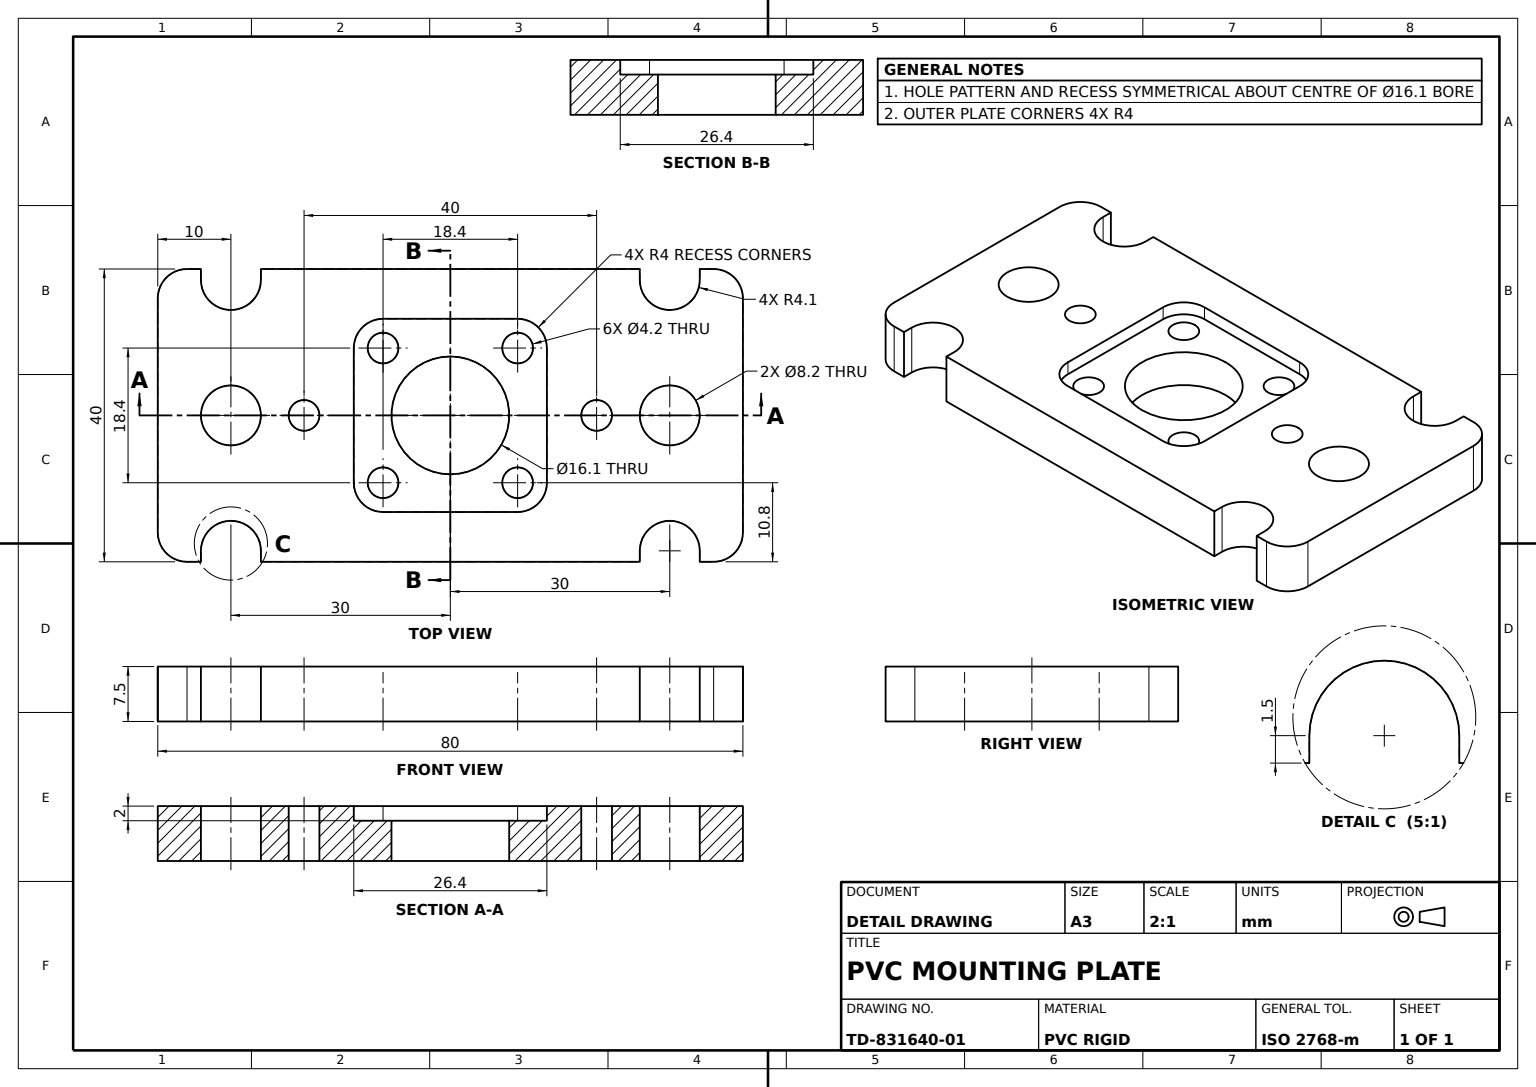
solid
v1 (-40,7.5,-16)
v2 (-40,0,-16)
e1 v1 v2 LINE
v3 (-36,7.5,-20)
e2 v3 v1 CIRCLE(AX(P(-36,7.5,-16),D(0,1,0),D(0,0,-1)),4)
v4 (-36,0,-20)
e3 v3 v4 LINE
e4 v4 v2 CIRCLE(AX(P(-36,0,-16),D(0,1,0),D(0,0,-1)),4)
face CYL(AX(P(-36,7.5,-16),D(0,-1,0),D(0,0,-1)),4) [-e1 -e2 e3 e4]
v5 (36,7.5,-20)
v6 (36,0,-20)
e5 v5 v6 LINE
v7 (40,7.5,-16)
e6 v7 v5 CIRCLE(AX(P(36,7.5,-16),D(0,1,0),D(0,0,1)),4)
v8 (40,0,-16)
e7 v7 v8 LINE
e8 v8 v6 CIRCLE(AX(P(36,0,-16),D(0,1,0),D(0,0,1)),4)
face CYL(AX(P(36,7.5,-16),D(0,-1,0),D(0,0,-1)),4) [-e5 -e6 e7 e8]
v9 (-20,7.5,2.1)
v10 (-20,7.5,-2.1)
e9 v9 v10 CIRCLE(AX(P(-20,7.5,0),D(0,1,0),D(0,0,1)),2.1)
v11 (-20,0,-2.1)
e10 v10 v11 LINE
v12 (-20,0,2.1)
e11 v12 v11 CIRCLE(AX(P(-20,0,0),D(0,1,0),D(0,0,1)),2.1)
e12 v9 v12 LINE
face CYL(AX(P(-20,7.5,0),D(0,-1,0),D(0,0,-1)),2.1) rev [e9 e10 -e11 -e12]
v13 (-9.2,0,-11.3)
v14 (-9.2,5.5,-11.3)
e13 v13 v14 LINE
v15 (-9.2,0,-7.1)
e14 v13 v15 CIRCLE(AX(P(-9.2,0,-9.2),D(0,-1,0),D(0,0,1)),2.1)
v16 (-9.2,5.5,-7.1)
e15 v15 v16 LINE
e16 v16 v14 CIRCLE(AX(P(-9.2,5.5,-9.2),D(0,1,0),D(0,0,1)),2.1)
face CYL(AX(P(-9.2,-0.001,-9.2),D(0,1,0),D(0,0,1)),2.1) rev [-e13 e14 e15 e16]
v17 (34.1,7.5,-18.5)
v18 (34.1,0,-18.5)
e17 v17 v18 LINE
v19 (25.9,0,-18.5)
e18 v18 v19 CIRCLE(AX(P(30,0,-18.5),D(0,-1,0),D(0,0,1)),4.1)
v20 (25.9,7.5,-18.5)
e19 v20 v19 LINE
e20 v17 v20 CIRCLE(AX(P(30,7.5,-18.5),D(0,-1,0),D(0,0,1)),4.1)
face CYL(AX(P(30,7.5,-18.5),D(0,-1,0),D(0,0,-1)),4.1) rev [e17 e18 -e19 -e20]
v21 (-9.2,0,7.1)
v22 (-9.2,5.5,7.1)
e21 v21 v22 LINE
v23 (-9.2,5.5,11.3)
e22 v22 v23 CIRCLE(AX(P(-9.2,5.5,9.2),D(0,1,0),D(0,0,-1)),2.1)
v24 (-9.2,0,11.3)
e23 v24 v23 LINE
e24 v24 v21 CIRCLE(AX(P(-9.2,0,9.2),D(0,-1,0),D(0,0,1)),2.1)
face CYL(AX(P(-9.2,-0.001,9.2),D(0,1,0),D(0,0,1)),2.1) rev [e21 e22 -e23 e24]
v25 (-34.1,7.5,18.5)
v26 (-34.1,0,18.5)
e25 v25 v26 LINE
v27 (-30,0,14.4)
e26 v26 v27 CIRCLE(AX(P(-30,0,18.5),D(0,-1,0),D(0,0,-1)),4.1)
v28 (-30,7.5,14.4)
e27 v28 v27 LINE
e28 v25 v28 CIRCLE(AX(P(-30,7.5,18.5),D(0,-1,0),D(0,0,-1)),4.1)
face CYL(AX(P(-30,7.5,18.5),D(0,-1,0),D(0,0,-1)),4.1) rev [e25 e26 -e27 -e28]
v29 (0,0,8.05)
v30 (0,5.5,8.05)
e29 v29 v30 LINE
v31 (0,5.5,-8.05)
e30 v30 v31 CIRCLE(AX(P(0,5.5,0),D(0,1,0),D(0,0,1)),8.05)
v32 (0,0,-8.05)
e31 v32 v31 LINE
e32 v32 v29 CIRCLE(AX(P(0,0,0),D(0,-1,0),D(0,0,1)),8.05)
face CYL(AX(P(0,-0.001,0),D(0,1,0),D(0,0,1)),8.05) rev [e29 e30 -e31 e32]
e33 v11 v12 CIRCLE(AX(P(-20,0,0),D(0,1,0),D(0,0,1)),2.1)
e34 v10 v9 CIRCLE(AX(P(-20,7.5,0),D(0,1,0),D(0,0,1)),2.1)
face CYL(AX(P(-20,7.5,0),D(0,-1,0),D(0,0,-1)),2.1) rev [-e33 -e10 e34 e12]
v33 (9.2,0,-11.3)
v34 (9.2,5.5,-11.3)
e35 v33 v34 LINE
v35 (9.2,5.5,-7.1)
e36 v34 v35 CIRCLE(AX(P(9.2,5.5,-9.2),D(0,1,0),D(0,0,-1)),2.1)
v36 (9.2,0,-7.1)
e37 v36 v35 LINE
e38 v36 v33 CIRCLE(AX(P(9.2,0,-9.2),D(0,-1,0),D(0,0,1)),2.1)
face CYL(AX(P(9.2,-0.001,-9.2),D(0,1,0),D(0,0,1)),2.1) rev [e35 e36 -e37 e38]
e39 v33 v36 CIRCLE(AX(P(9.2,0,-9.2),D(0,-1,0),D(0,0,1)),2.1)
e40 v35 v34 CIRCLE(AX(P(9.2,5.5,-9.2),D(0,1,0),D(0,0,-1)),2.1)
face CYL(AX(P(9.2,-0.001,-9.2),D(0,1,0),D(0,0,1)),2.1) rev [-e35 e39 e37 e40]
v37 (36,7.5,20)
v38 (36,0,20)
e41 v37 v38 LINE
v39 (34.1,7.5,20)
e42 v39 v37 LINE
v40 (34.1,0,20)
e43 v39 v40 LINE
e44 v40 v38 LINE
face PLANE(AX(P(34.1,7.5,20),D(0,0,-1),D(-1,0,0))) rev [-e41 -e42 e43 e44]
v41 (-9.2,5.5,-13.2)
v42 (-9.2,7.5,-13.2)
e45 v41 v42 LINE
v43 (-13.2,7.5,-9.2)
e46 v42 v43 CIRCLE(AX(P(-9.2,7.5,-9.2),D(0,1,0),D(0,0,1)),4)
v44 (-13.2,5.5,-9.2)
e47 v44 v43 LINE
e48 v41 v44 CIRCLE(AX(P(-9.2,5.5,-9.2),D(0,1,0),D(0,0,1)),4)
face CYL(AX(P(-9.2,5.5,-9.2),D(0,1,0),D(0,0,1)),4) rev [e45 e46 -e47 -e48]
v45 (9.2,0,7.1)
v46 (9.2,5.5,7.1)
e49 v45 v46 LINE
v47 (9.2,0,11.3)
e50 v45 v47 CIRCLE(AX(P(9.2,0,9.2),D(0,-1,0),D(0,0,1)),2.1)
v48 (9.2,5.5,11.3)
e51 v47 v48 LINE
e52 v48 v46 CIRCLE(AX(P(9.2,5.5,9.2),D(0,1,0),D(0,0,1)),2.1)
face CYL(AX(P(9.2,-0.001,9.2),D(0,1,0),D(0,0,1)),2.1) rev [-e49 e50 e51 e52]
v49 (30,0,4.1)
v50 (30,0,-4.1)
e53 v49 v50 CIRCLE(AX(P(30,0,0),D(0,1,0),D(0,0,-1)),4.1)
v51 (30,7.5,4.1)
e54 v51 v49 LINE
v52 (30,7.5,-4.1)
e55 v51 v52 CIRCLE(AX(P(30,7.5,0),D(0,1,0),D(0,0,-1)),4.1)
e56 v52 v50 LINE
face CYL(AX(P(30,7.5,0),D(0,-1,0),D(0,0,-1)),4.1) rev [-e53 -e54 e55 e56]
e57 v14 v16 CIRCLE(AX(P(-9.2,5.5,-9.2),D(0,1,0),D(0,0,1)),2.1)
e58 v15 v13 CIRCLE(AX(P(-9.2,0,-9.2),D(0,-1,0),D(0,0,1)),2.1)
face CYL(AX(P(-9.2,-0.001,-9.2),D(0,1,0),D(0,0,1)),2.1) rev [e57 -e15 e58 e13]
v53 (9.2,5.5,13.2)
v54 (9.2,7.5,13.2)
e59 v53 v54 LINE
v55 (-9.2,5.5,13.2)
e60 v55 v53 LINE
v56 (-9.2,7.5,13.2)
e61 v55 v56 LINE
e62 v56 v54 LINE
face PLANE(AX(P(-9.2,5.5,13.2),D(0,0,1),D(1,0,0))) rev [-e59 -e60 e61 e62]
v57 (-30,7.5,-4.1)
v58 (-30,0,-4.1)
e63 v57 v58 LINE
v59 (-30,7.5,4.1)
e64 v57 v59 CIRCLE(AX(P(-30,7.5,0),D(0,1,0),D(0,0,1)),4.1)
v60 (-30,0,4.1)
e65 v59 v60 LINE
e66 v58 v60 CIRCLE(AX(P(-30,0,0),D(0,1,0),D(0,0,1)),4.1)
face CYL(AX(P(-30,7.5,0),D(0,-1,0),D(0,0,-1)),4.1) rev [-e63 e64 e65 -e66]
e67 v50 v49 CIRCLE(AX(P(30,0,0),D(0,1,0),D(0,0,-1)),4.1)
e68 v52 v51 CIRCLE(AX(P(30,7.5,0),D(0,1,0),D(0,0,-1)),4.1)
face CYL(AX(P(30,7.5,0),D(0,-1,0),D(0,0,-1)),4.1) rev [-e67 -e56 e68 e54]
v61 (-25.9,7.5,-18.5)
v62 (-25.9,0,-18.5)
e69 v61 v62 LINE
v63 (-25.9,7.5,-20)
e70 v63 v61 LINE
v64 (-25.9,0,-20)
e71 v63 v64 LINE
e72 v64 v62 LINE
face PLANE(AX(P(-25.9,7.5,-18.5),D(1,0,0),D(0,0,-1))) rev [-e69 -e70 e71 e72]
v65 (34.1,0,-20)
e73 v6 v65 LINE
v66 (34.1,7.5,-20)
e74 v66 v65 LINE
e75 v5 v66 LINE
face PLANE(AX(P(34.1,7.5,-20),D(0,0,1),D(1,0,0))) rev [e5 e73 -e74 -e75]
v67 (20,0,-2.1)
v68 (20,0,2.1)
e76 v67 v68 CIRCLE(AX(P(20,0,0),D(0,1,0),D(0,0,-1)),2.1)
v69 (20,7.5,-2.1)
e77 v69 v67 LINE
v70 (20,7.5,2.1)
e78 v69 v70 CIRCLE(AX(P(20,7.5,0),D(0,1,0),D(0,0,-1)),2.1)
e79 v70 v68 LINE
face CYL(AX(P(20,7.5,0),D(0,-1,0),D(0,0,-1)),2.1) rev [-e76 -e77 e78 e79]
v71 (-34.1,7.5,-20)
e80 v71 v3 LINE
v72 (-40,7.5,16)
e81 v1 v72 LINE
v73 (-36,7.5,20)
e82 v72 v73 CIRCLE(AX(P(-36,7.5,16),D(0,1,0),D(0,0,1)),4)
v74 (-34.1,7.5,20)
e83 v73 v74 LINE
e84 v74 v25 LINE
v75 (-25.9,7.5,18.5)
e85 v28 v75 CIRCLE(AX(P(-30,7.5,18.5),D(0,-1,0),D(0,0,-1)),4.1)
v76 (-25.9,7.5,20)
e86 v75 v76 LINE
v77 (25.9,7.5,20)
e87 v76 v77 LINE
v78 (25.9,7.5,18.5)
e88 v77 v78 LINE
v79 (30,7.5,14.4)
e89 v78 v79 CIRCLE(AX(P(30,7.5,18.5),D(0,-1,0),D(0,0,-1)),4.1)
v80 (34.1,7.5,18.5)
e90 v79 v80 CIRCLE(AX(P(30,7.5,18.5),D(0,-1,0),D(0,0,-1)),4.1)
e91 v80 v39 LINE
v81 (40,7.5,16)
e92 v37 v81 CIRCLE(AX(P(36,7.5,16),D(0,1,0),D(0,0,-1)),4)
e93 v81 v7 LINE
e94 v66 v17 LINE
v82 (25.9,7.5,-20)
e95 v20 v82 LINE
e96 v82 v63 LINE
v83 (-34.1,7.5,-18.5)
e97 v61 v83 CIRCLE(AX(P(-30,7.5,-18.5),D(0,-1,0),D(0,0,1)),4.1)
e98 v83 v71 LINE
e99 v70 v69 CIRCLE(AX(P(20,7.5,0),D(0,1,0),D(0,0,-1)),2.1)
v84 (13.2,7.5,9.2)
v85 (13.2,7.5,-9.2)
e100 v84 v85 LINE
e101 v54 v84 CIRCLE(AX(P(9.2,7.5,9.2),D(0,1,0),D(0,0,1)),4)
v86 (-13.2,7.5,9.2)
e102 v86 v56 CIRCLE(AX(P(-9.2,7.5,9.2),D(0,1,0),D(0,0,1)),4)
e103 v43 v86 LINE
v87 (9.2,7.5,-13.2)
e104 v87 v42 LINE
e105 v85 v87 CIRCLE(AX(P(9.2,7.5,-9.2),D(0,1,0),D(0,0,1)),4)
e106 v59 v57 CIRCLE(AX(P(-30,7.5,0),D(0,1,0),D(0,0,1)),4.1)
face PLANE(AX(P(36,7.5,-16),D(0,1,0),D(0,0,1))) [e80 e2 e81 e82 e83 e84 e28 e85 e86 e87 e88 e89 e90 e91 e42 e92 e93 e6 e75 e94 e20 e95 e96 e70 e97 e98] [-e99 -e78] [-e100 -e101 -e62 -e102 -e103 -e46 -e104 -e105] [-e9 -e34] [-e55 -e68] [-e106 -e64]
e107 v29 v32 CIRCLE(AX(P(0,0,0),D(0,-1,0),D(0,0,1)),8.05)
e108 v47 v45 CIRCLE(AX(P(9.2,0,9.2),D(0,-1,0),D(0,0,1)),2.1)
e109 v21 v24 CIRCLE(AX(P(-9.2,0,9.2),D(0,-1,0),D(0,0,1)),2.1)
e110 v68 v67 CIRCLE(AX(P(20,0,0),D(0,1,0),D(0,0,-1)),2.1)
v88 (-40,0,16)
v89 (-36,0,20)
e111 v88 v89 CIRCLE(AX(P(-36,0,16),D(0,1,0),D(0,0,1)),4)
e112 v2 v88 LINE
v90 (-34.1,0,-20)
e113 v90 v4 LINE
v91 (-34.1,0,-18.5)
e114 v91 v90 LINE
e115 v62 v91 CIRCLE(AX(P(-30,0,-18.5),D(0,-1,0),D(0,0,1)),4.1)
v92 (25.9,0,-20)
e116 v92 v64 LINE
e117 v19 v92 LINE
e118 v65 v18 LINE
v93 (40,0,16)
e119 v93 v8 LINE
e120 v38 v93 CIRCLE(AX(P(36,0,16),D(0,1,0),D(0,0,-1)),4)
v94 (34.1,0,18.5)
e121 v94 v40 LINE
v95 (30,0,14.4)
e122 v95 v94 CIRCLE(AX(P(30,0,18.5),D(0,-1,0),D(0,0,-1)),4.1)
v96 (25.9,0,18.5)
e123 v96 v95 CIRCLE(AX(P(30,0,18.5),D(0,-1,0),D(0,0,-1)),4.1)
v97 (25.9,0,20)
e124 v97 v96 LINE
v98 (-25.9,0,20)
e125 v98 v97 LINE
v99 (-25.9,0,18.5)
e126 v99 v98 LINE
e127 v27 v99 CIRCLE(AX(P(-30,0,18.5),D(0,-1,0),D(0,0,-1)),4.1)
v100 (-34.1,0,20)
e128 v100 v26 LINE
e129 v89 v100 LINE
e130 v60 v58 CIRCLE(AX(P(-30,0,0),D(0,1,0),D(0,0,1)),4.1)
face PLANE(AX(P(36,0,-16),D(0,1,0),D(0,0,1))) rev [-e107 -e32] [e53 e67] [-e50 -e108] [-e24 -e109] [e76 e110] [-e38 -e39] [-e111 -e112 -e4 -e113 -e114 -e115 -e72 -e116 -e117 -e18 -e118 -e73 -e8 -e119 -e120 -e44 -e121 -e122 -e123 -e124 -e125 -e126 -e127 -e26 -e128 -e129] [e11 e33] [-e58 -e14] [e130 e66]
e131 v71 v90 LINE
face PLANE(AX(P(-36,7.5,-20),D(0,0,1),D(1,0,0))) rev [-e80 e131 e113 -e3]
v101 (9.2,5.5,-13.2)
e132 v101 v87 LINE
e133 v101 v41 LINE
face PLANE(AX(P(-9.2,5.5,-13.2),D(0,0,-1),D(-1,0,0))) rev [e132 e104 -e45 -e133]
e134 v80 v94 LINE
e135 v79 v95 LINE
face CYL(AX(P(30,7.5,18.5),D(0,-1,0),D(0,0,-1)),4.1) rev [e122 -e134 -e90 e135]
e136 v78 v96 LINE
face CYL(AX(P(30,7.5,18.5),D(0,-1,0),D(0,0,-1)),4.1) rev [e123 -e135 -e89 e136]
e137 v31 v30 CIRCLE(AX(P(0,5.5,0),D(0,1,0),D(0,0,1)),8.05)
v102 (-13.2,5.5,9.2)
e138 v44 v102 LINE
e139 v102 v55 CIRCLE(AX(P(-9.2,5.5,9.2),D(0,1,0),D(0,0,1)),4)
v103 (13.2,5.5,9.2)
e140 v53 v103 CIRCLE(AX(P(9.2,5.5,9.2),D(0,1,0),D(0,0,1)),4)
v104 (13.2,5.5,-9.2)
e141 v103 v104 LINE
e142 v104 v101 CIRCLE(AX(P(9.2,5.5,-9.2),D(0,1,0),D(0,0,1)),4)
e143 v23 v22 CIRCLE(AX(P(-9.2,5.5,9.2),D(0,1,0),D(0,0,-1)),2.1)
e144 v46 v48 CIRCLE(AX(P(9.2,5.5,9.2),D(0,1,0),D(0,0,1)),2.1)
face PLANE(AX(P(-9.2,5.5,9.2),D(0,1,0),D(0,0,1))) [-e30 -e137] [e48 e138 e139 e60 e140 e141 e142 e133] [-e22 -e143] [-e52 -e144] [-e16 -e57] [-e40 -e36]
face CYL(AX(P(-30,7.5,0),D(0,-1,0),D(0,0,-1)),4.1) rev [-e65 e106 e63 -e130]
e145 v81 v93 LINE
face CYL(AX(P(36,7.5,16),D(0,-1,0),D(0,0,-1)),4) [e41 e120 -e145 -e92]
face CYL(AX(P(20,7.5,0),D(0,-1,0),D(0,0,-1)),2.1) rev [-e110 -e79 e99 e77]
e146 v82 v92 LINE
face PLANE(AX(P(-25.9,7.5,-20),D(0,0,1),D(1,0,0))) rev [-e71 -e96 e146 e116]
face CYL(AX(P(0,-0.001,0),D(0,1,0),D(0,0,1)),8.05) rev [e137 -e29 e107 e31]
e147 v75 v99 LINE
e148 v76 v98 LINE
face PLANE(AX(P(-25.9,7.5,18.5),D(1,0,0),D(0,0,-1))) rev [-e86 e147 e126 -e148]
face PLANE(AX(P(34.1,7.5,-18.5),D(1,0,0),D(0,0,-1))) rev [e118 -e17 -e94 e74]
face PLANE(AX(P(40,7.5,16),D(-1,0,0),D(0,0,1))) rev [e145 e119 -e7 -e93]
e149 v83 v91 LINE
face PLANE(AX(P(-34.1,7.5,-20),D(-1,0,0),D(0,0,1))) rev [-e98 e149 e114 -e131]
face PLANE(AX(P(25.9,7.5,-20),D(-1,0,0),D(0,0,1))) rev [-e95 e19 e117 -e146]
face CYL(AX(P(9.2,-0.001,9.2),D(0,1,0),D(0,0,1)),2.1) rev [e144 -e51 e108 e49]
e150 v72 v88 LINE
e151 v73 v89 LINE
face CYL(AX(P(-36,7.5,16),D(0,-1,0),D(0,0,-1)),4) [-e82 e150 e111 -e151]
face PLANE(AX(P(34.1,7.5,18.5),D(1,0,0),D(0,0,-1))) rev [-e91 e134 e121 -e43]
e152 v103 v84 LINE
face CYL(AX(P(9.2,5.5,9.2),D(0,1,0),D(0,0,1)),4) rev [-e140 e59 e101 -e152]
e153 v77 v97 LINE
face PLANE(AX(P(25.9,7.5,20),D(-1,0,0),D(0,0,1))) rev [e153 e124 -e136 -e88]
e154 v74 v100 LINE
face PLANE(AX(P(-34.1,7.5,20),D(-1,0,0),D(0,0,1))) rev [-e84 e154 e128 -e25]
face PLANE(AX(P(-40,7.5,16),D(1,0,0),D(0,0,-1))) rev [-e81 e1 e112 -e150]
face CYL(AX(P(-9.2,-0.001,9.2),D(0,1,0),D(0,0,1)),2.1) rev [e109 e23 e143 -e21]
face CYL(AX(P(-30,7.5,-18.5),D(0,-1,0),D(0,0,-1)),4.1) rev [e115 -e149 -e97 e69]
e155 v102 v86 LINE
face PLANE(AX(P(-13.2,5.5,9.2),D(-1,0,0),D(0,0,1))) rev [-e155 -e138 e47 e103]
e156 v104 v85 LINE
face PLANE(AX(P(13.2,5.5,9.2),D(1,0,0),D(0,0,-1))) rev [-e141 e152 e100 -e156]
face CYL(AX(P(-9.2,5.5,9.2),D(0,1,0),D(0,0,1)),4) rev [e102 -e61 -e139 e155]
face CYL(AX(P(9.2,5.5,-9.2),D(0,1,0),D(0,0,1)),4) rev [-e132 -e142 e156 e105]
face PLANE(AX(P(-25.9,7.5,20),D(0,0,-1),D(-1,0,0))) rev [-e87 e148 e125 -e153]
face CYL(AX(P(-30,7.5,18.5),D(0,-1,0),D(0,0,-1)),4.1) rev [e127 -e147 -e85 e27]
face PLANE(AX(P(-36,7.5,20),D(0,0,-1),D(-1,0,0))) rev [e151 e129 -e154 -e83]
